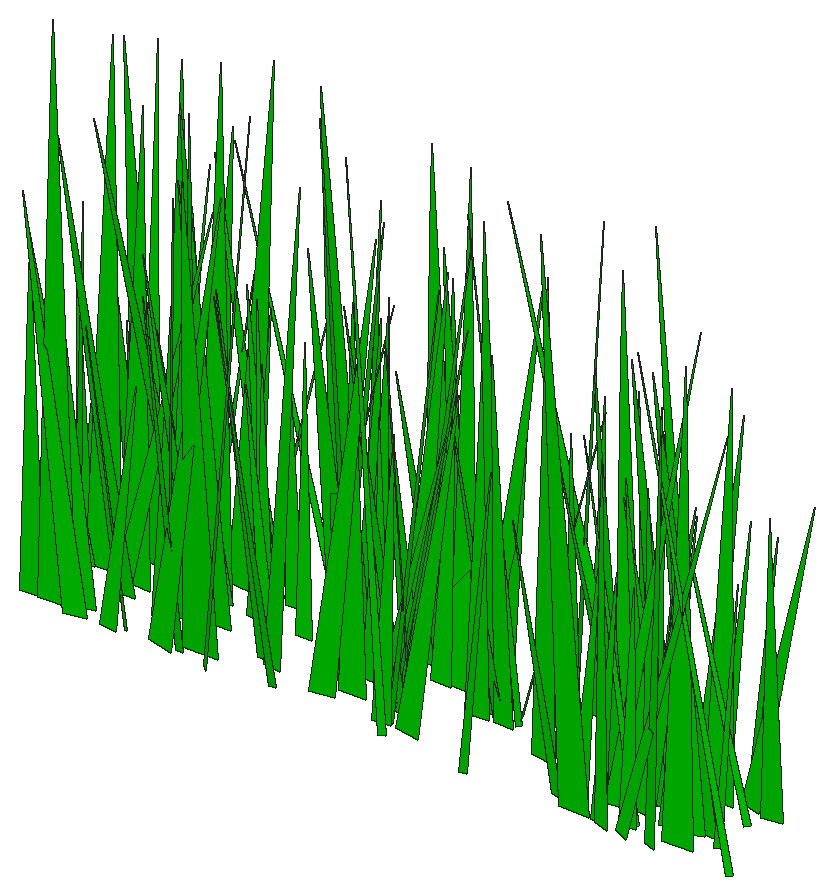
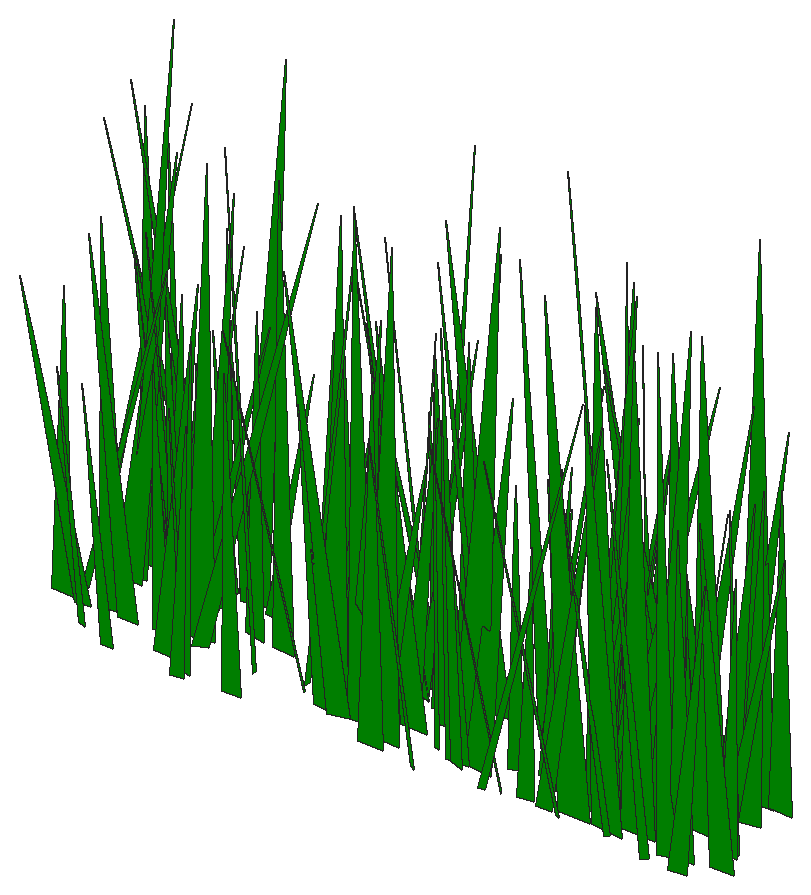
# SketchUp Ruby script. Lengths in inches.
U = 1.inch
M = Sketchup.active_model
def pt(a) = Geom::Point3d.new(a.map { |v| v * U })
def face(e, loops, mat)
  f = e.add_face(loops[0].map { |a| pt(a) })
  loops[1..].each { |l| e.add_face(l.map { |a| pt(a) }).erase! }
  f.material = f.back_material = mat if mat
  f
end
# faces: each face lists its corners as indices into pts; further lists are holes
def faces(e, pts, list, mat = nil) = list.each { |f| face(e, (f[0].is_a?(Array) ? f : [f]).map { |l| l.map { |i| pts[i] } }, mat) }
# xy, xz, yz: faces in a plane at the given z, y or x. An outline is a flat list of corners, or four numbers for a rectangle; further outlines are holes
def ring(l) = l.size == 4 ? [[l[0], l[1]], [l[2], l[1]], [l[2], l[3]], [l[0], l[3]]] : l.each_slice(2).to_a
def flat(e, list, mat, &to3) = list.each { |f| face(e, (f[0].is_a?(Array) ? f : [f]).map { |l| ring(l).map { |u, v| to3.(u, v) } }, mat) }
def xy(e, z, list, mat = nil) = flat(e, list, mat) { |x, y| [x, y, z] }
def xz(e, y, list, mat = nil) = flat(e, list, mat) { |x, z| [x, y, z] }
def yz(e, x, list, mat = nil) = flat(e, list, mat) { |y, z| [x, y, z] }
def lines(e, pts, list) = list.each { |a, b| e.add_line(pt(pts[a]), pt(pts[b])) }
# prism: a flat outline (further loops are holes) pulled along v
def prism(e, loops, v, mat = nil)
  f = face(e, loops, mat); d = Geom::Vector3d.new(v.map { |x| x * U })
  f.pushpull(f.normal.samedirection?(d) ? d.length : -d.length)
end
def box(e, o, s, mat = nil) = prism(e, [[o, [o[0] + s[0], o[1], o[2]], [o[0] + s[0], o[1] + s[1], o[2]], [o[0], o[1] + s[1], o[2]]]], [0, 0, s[2]], mat)
def at(x, y, z, deg = 0) = Geom::Transformation.translation(pt([x, y, z])) * Geom::Transformation.rotation(ORIGIN, Z_AXIS, deg.degrees)
def axes(o, x, y, z) = Geom::Transformation.new([*x, 0, *y, 0, *z, 0, *pt(o).to_a, 1])
def part(name) = M.definitions.add(name)
# library, detail: a bought-in or finely detailed component or shape, given as its bounding box
def library(name, o, s) = part(name).tap { |d| box(d.entities, o, s) }
def detail(e, o, s) = box(e.add_group.entities, o, s)
def put(e, d, t, mat = nil) = e.add_instance(d, t).tap { |i| i.material = mat if mat }
def group(e, t, mat = nil) = e.add_group.tap { |g| g.transformation = t; g.material = mat if mat }.entities
root = M.entities
M.materials.add("[Color G06]").color = [0, 204, 0]
c1 = part("fur_instance\#9")
p = [[0.8125,0,1.79],[0.67,-0.02,1.48],[0,-0.11,0],[0,0.11,0]]
faces(c1.entities,p,[[0,1,2,3]])
put(root,c1,axes([40.12,23.45,4.28],[-2.85245,0.30884,0.19412],[2.21845,0.39741,0.18428],[0.02687,-0.02469,5.39428]),"[Color G06]")
put(root,c1,axes([39.12,24.88,4.28],[0.44587,0.55522,0.43094],[3.99144,-0.06132,-0.15003],[0.06794,-0.04151,5.9861]),"[Color G06]")
put(root,c1,axes([39.53,24.09,4.28],[-1.47784,0.3217,1.91072],[2.58234,0.21807,0.24368],[0.53687,-0.16338,4.08752]),"[Color G06]")
put(root,c1,axes([39.44,23.875,4.28],[3.17546,0.17629,2.14393],[1.36851,-0.48036,0.0098],[-1.33536,-0.07307,5.10824]),"[Color G06]")
put(root,c1,axes([40.04,25.73,4.28],[-1.25995,-0.44632,0.01521],[-3.19526,0.17548,0.29333],[0.18635,-0.00871,5.13257]),"[Color G06]")
put(root,c1,axes([39.9375,21.28,4.28],[-0.04363,0.5128,0.83195],[3.71653,0.00302,0.22126],[-0.14312,-0.0778,5.49207]),"[Color G06]")
put(root,c1,axes([40.17,22.35,4.28],[-1.71212,0.49575,0.61747],[3.56156,0.2423,-0.28791],[0.35356,-0.04012,5.89045]),"[Color G06]")
put(root,c1,axes([40.41,25.09,4.28],[-0.2839,0.54186,0.38757],[3.8943,0.03985,-0.02844],[0.03791,-0.03587,5.82309]),"[Color G06]")
put(root,c1,axes([40.58,23.59,4.28],[0.53286,0.81064,0.81045],[5.83043,-0.07789,0.3865],[-0.30808,-0.07192,8.71631]),"[Color G06]")
put(root,c1,axes([41.58,21.08,4.28],[-2.68815,0.49164,0.54662],[3.54364,0.37426,0.25796],[0.08386,-0.05517,6.62131]),"[Color G06]")
put(root,c1,axes([40.51,24.95,4.28],[2.30914,0.16016,1.70391],[1.34151,-0.34437,-0.34264],[-0.9051,-0.10181,3.83924]),"[Color G06]")
put(root,c1,axes([40.79,21.3,4.28],[-1.94564,0.73172,3.76087],[5.76334,0.29356,0.09892],[0.80672,-0.3325,8.36373]),"[Color G06]")
put(root,c1,axes([41.96,22.81,4.28],[-3.36752,-0.46867,1.06526],[-3.42077,0.47034,-0.38423],[0.32011,0.09577,7.10044]),"[Color G06]")
put(root,c1,axes([41.54,21.58,4.28],[-1.2926,0.44884,0.766],[3.25907,0.1771,0.36367],[-0.03773,-0.07894,5.17128]),"[Color G06]")
put(root,c1,axes([40.85,25.21,4.28],[-4.35201,0.29976,3.63094],[2.42253,0.67732,0.06246],[2.15741,-0.15587,7.25434]),"[Color G06]")
put(root,c1,axes([41.42,24.6,4.28],[-1.33979,-0.77155,1.33619],[-5.5985,0.19029,0.08295],[0.26499,0.11932,8.50806]),"[Color G06]")
put(root,c1,axes([41.77,23.53,4.28],[2.11226,0.16366,1.89723],[1.30087,-0.33453,0.07983],[-1.13866,-0.0786,3.61063]),"[Color G06]")
put(root,c1,axes([41.76,23.4,4.28],[1.30253,-0.60335,3.45497],[-4.88502,-0.19005,0.30115],[-0.44897,0.31746,6.74666]),"[Color G06]")
put(root,c1,axes([41.25,25.7,4.28],[3.97968,-0.126,1.6751],[-0.96593,-0.57436,0.16321],[-1.06751,0.04999,6.09712]),"[Color G06]")
put(root,c1,axes([42.23,24.73,4.28],[-0.08104,0.74769,1.61282],[5.4693,0.01021,0.06995],[-0.03143,-0.15056,8.01433]),"[Color G06]")
put(root,c1,axes([43.875,23.49,4.28],[-4.07687,-0.46189,0.12276],[-3.31329,0.56845,-0.09246],[0.02473,0.01392,7.85025]),"[Color G06]")
put(root,c1,axes([43.18,21.29,4.28],[-3.05858,-0.00912,0.90232],[-0.11198,0.43336,-0.34468],[0.59685,0.03457,4.55931]),"[Color G06]")
put(root,c1,axes([43.03,25.13,4.28],[0.87527,0.70528,0.00052],[5.05312,-0.12194,0.32835],[-0.21654,0.00518,7.66451]),"[Color G06]")
put(root,c1,axes([42.7,21.1,4.28],[1.56069,-0.31586,0.71684],[-2.3132,-0.21616,0.30827],[-0.09896,0.07148,4.09956]),"[Color G06]")
put(root,c1,axes([41.72,22.92,4.28],[4.18376,-0.32444,0.21167],[-2.33055,-0.58297,0.24962],[-0.04249,0.02996,7.15043]),"[Color G06]")
put(root,c1,axes([44.04,24.15,4.28],[-3.04206,-0.4363,1.2577],[-3.15653,0.43539,0.2961],[0.73067,0.06443,6.51543]),"[Color G06]")
put(root,c1,axes([43.47,22.42,4.28],[1.61179,0.3871,1.23984],[2.83559,-0.23793,0.29931],[-0.59461,-0.08536,4.78818]),"[Color G06]")
put(root,c1,axes([44.375,24.09,4.28],[-1.61041,0.32888,0.22325],[2.36127,0.22291,0.32439],[-0.0955,-0.03424,4.25592]),"[Color G06]")
put(root,c1,axes([42.88,25.32,4.28],[3.32389,-0.08797,0.96952],[-0.64275,-0.47193,0.00294],[-0.63694,0.01714,5.05649]),"[Color G06]")
put(root,c1,axes([43.67,24.47,4.28],[-0.49846,0.74899,2.28351],[5.57775,0.07713,-0.18644],[0.27024,-0.21041,8.06001]),"[Color G06]")
put(root,c1,axes([44.63,22.85,4.28],[-2.74102,-0.16449,0.75095],[-1.23185,0.38373,-0.38792],[0.35573,0.06131,4.44303]),"[Color G06]")
put(root,c1,axes([43.84,22.76,4.28],[-1.16878,0.43335,2.18051],[3.37735,0.18371,-0.15035],[0.61619,-0.18494,4.96]),"[Color G06]")
put(root,c1,axes([44.93,22.38,4.28],[-2.90629,-0.38229,0.67175],[-2.76421,0.40699,-0.10738],[0.27729,0.05033,5.97027]),"[Color G06]")
put(root,c1,axes([45.21,25.22,4.28],[-3.96426,0.29588,1.18407],[2.18573,0.55814,0.3245],[0.59363,-0.07918,6.71235]),"[Color G06]")
put(root,c1,axes([44.68,23.26,4.28],[-3.70896,0.24437,1.80022],[1.75941,0.54231,-0.35953],[1.19429,-0.04002,6.12038]),"[Color G06]")
put(root,c1,axes([44.23,21.83,4.28],[-4.11597,-0.09811,2.95033],[-0.72754,0.63585,0.16175],[1.96532,0.02991,6.23875]),"[Color G06]")
put(root,c1,axes([44.93,23.04,4.28],[-2.52644,-0.63889,2.27151],[-4.80201,0.35702,-0.39511],[0.49189,0.20389,7.80968]),"[Color G06]")
put(root,c1,axes([45.01,21.31,4.28],[-3.27274,-0.18283,1.3921],[-1.39777,0.46901,-0.26419],[0.79555,0.07191,5.26266]),"[Color G06]")
put(root,c1,axes([44.25,25.07,4.28],[1.85243,0.73626,1.88589],[5.41345,-0.26442,-0.0193],[-0.40525,-0.16664,8.36277]),"[Color G06]")
put(root,c1,axes([44.79,22.05,4.28],[-4.66954,-0.25669,3.43881],[-2.07416,0.71337,-0.17439],[2.0929,0.13429,7.49963]),"[Color G06]")
put(root,c1,axes([44.42,21.21,4.28],[3.18828,0.53718,1.30508],[3.93312,-0.44618,-0.36599],[-0.36458,-0.11579,7.46465]),"[Color G06]")
put(root,c1,axes([47.26,25.42,4.28],[-4.91589,0.08106,0.36127],[0.59262,0.68538,0.34647],[0.21253,-0.03609,7.39023]),"[Color G06]")
put(root,c1,axes([45.53,21.57,4.28],[-0.16652,-0.77235,0.00783],[-5.53873,0.02322,0.00849],[0.00583,0.00071,8.28177]),"[Color G06]")
put(root,c1,axes([45.43,23.98,4.28],[2.38175,0.29892,1.42613],[2.21462,-0.34903,0.14227],[-0.77537,-0.07868,4.78705]),"[Color G06]")
put(root,c1,axes([46.21,23.76,4.28],[-2.2505,0.37025,1.19816],[2.7297,0.32117,0.05201],[0.49108,-0.08849,5.20173]),"[Color G06]")
put(root,c1,axes([45.94,25.11,4.28],[-1.16822,0.34539,1.05232],[2.55153,0.1698,-0.07516],[0.34726,-0.0857,4.09233]),"[Color G06]")
put(root,c1,axes([46.03,23.72,4.28],[-2.25727,0.32442,1.67701],[2.43983,0.33601,-0.13146],[0.84786,-0.10322,4.84301]),"[Color G06]")
put(root,c1,axes([44.64,25.33,4.28],[3.68565,0.12271,0.38905],[0.88593,-0.51496,-0.08893],[-0.23931,-0.01652,5.66261]),"[Color G06]")
put(root,c1,axes([47,22.39,4.28],[-3.36731,-0.21704,1.2149],[-1.62701,0.47786,-0.26638],[0.66045,0.0706,5.53792]),"[Color G06]")
put(root,c1,axes([46.59,23.0625,4.28],[0.27,-0.39209,1.36575],[-2.95249,-0.04246,-0.09639],[-0.1548,0.12591,4.22064]),"[Color G06]")
put(root,c1,axes([47.17,22.54,4.28],[-1.66988,0.31077,0.77043],[2.27575,0.23469,0.14356],[0.23075,-0.06566,4.1596]),"[Color G06]")
put(root,c1,axes([46.14,21.02,4.28],[5.69893,0.13608,2.64151],[1.04334,-0.83037,-0.11401],[-1.72843,-0.05256,8.64069]),"[Color G06]")
put(root,c1,axes([47.17,24,4.28],[1.91114,-0.27734,2.13718],[-2.2855,-0.29289,0.19915],[-0.88141,0.15811,4.11762]),"[Color G06]")
put(root,c1,axes([48.2,21.34,4.28],[-3.70295,-0.19382,1.03201],[-1.44498,0.52145,-0.33108],[0.56642,0.06314,5.90211]),"[Color G06]")
put(root,c1,axes([48.01,24.65,4.28],[-0.75998,-0.60579,0.19153],[-4.34378,0.10527,-0.25174],[-0.14392,0.02164,6.58663]),"[Color G06]")
put(root,c1,axes([47.55,22.14,4.28],[3.93587,0.41903,2.29981],[3.11444,-0.57787,0.18901],[-1.30302,-0.11549,7.3985]),"[Color G06]")
put(root,c1,axes([46.74,25.22,4.28],[3.75999,0.04929,0.42335],[0.34247,-0.52549,0.23363],[-0.29645,0.01807,5.63951]),"[Color G06]")
put(root,c1,axes([48.37,24.6,4.28],[-1.0832,-0.83788,1.06205],[-6.04963,0.15172,-0.03277],[0.10434,0.09806,9.12507]),"[Color G06]")
put(root,c1,axes([48.7,24.08,4.28],[-5.04094,-0.22111,2.62842],[-1.59717,0.74333,0.34092],[1.74818,0.04154,7.89062]),"[Color G06]")
put(root,c1,axes([48.65,24.82,4.28],[3.86213,0.30249,2.41646],[2.25592,-0.57698,0.24307],[-1.49351,-0.08929,6.61595]),"[Color G06]")
put(root,c1,axes([48.72,24.68,4.28],[1.23239,-0.48642,0.7673],[-3.5235,-0.17266,0.06723],[-0.12819,0.06961,5.52885]),"[Color G06]")
put(root,c1,axes([49.66,24.4,4.28],[-3.31285,-0.15227,2.41291],[-1.12798,0.51185,0.25122],[1.5895,0.04586,5.20728]),"[Color G06]")
put(root,c1,axes([49.14,23.02,4.28],[4.5547,0.22077,2.01328],[1.70523,-0.65555,-0.35945],[-1.18881,-0.09449,7.19788]),"[Color G06]")
put(root,c1,axes([50.17,22.34,4.28],[-0.06874,0.5647,1.44172],[4.1625,0.00737,0.11174],[-0.06047,-0.13465,6.05232]),"[Color G06]")
put(root,c1,axes([49.52,25.6875,4.28],[3.28467,0.11231,1.00551],[0.81818,-0.46711,0.02345],[-0.65722,-0.02018,5.05456]),"[Color G06]")
put(root,c1,axes([50.21,23.25,4.28],[1.3316,-0.52058,1.27764],[-3.82125,-0.18904,0.04802],[-0.25623,0.11381,5.92367]),"[Color G06]")
put(root,c1,axes([49.5,21.88,4.28],[3.817,-0.50031,1.12969],[-3.6229,-0.53805,-0.0299],[-0.56459,0.07014,7.82932]),"[Color G06]")
put(root,c1,axes([51.41,24.79,4.28],[-1.73515,-0.40131,0.02022],[-2.87789,0.24195,-0.02453],[-0.00707,0.0028,5.02244]),"[Color G06]")
put(root,c1,axes([51.23,23.65,4.28],[-0.85631,-0.47007,0.62233],[-3.39621,0.1176,-0.23426],[-0.05059,0.06164,5.19289]),"[Color G06]")
put(root,c1,axes([50.99,22.61,4.28],[-1.49738,0.34444,1.11468],[2.52223,0.22075,-0.26744],[0.54392,-0.0754,4.30878]),"[Color G06]")
put(root,c1,axes([51.85,22.35,4.28],[-3.52163,-0.30445,1.11288],[-2.244,0.49604,-0.27293],[0.53448,0.07665,6.18675]),"[Color G06]")
put(root,c1,axes([51.16,24.99,4.28],[-0.28699,0.73119,2.39369],[5.48041,0.03181,0.35136],[-0.15798,-0.22465,7.84073]),"[Color G06]")
put(root,c1,axes([51.22,25.42,4.28],[-0.39201,0.55416,1.30054],[4.06789,0.05494,0.04973],[0.05153,-0.12122,5.96814]),"[Color G06]")
put(root,c1,axes([50.85,23.94,4.28],[1.48248,0.60516,0.65009],[4.3605,-0.207,-0.07612],[-0.09219,-0.0597,6.85363]),"[Color G06]")
put(root,c1,axes([52.17,21.11,4.28],[-5.64778,0.07935,2.74293],[0.54179,0.82809,-0.26007],[1.84349,-0.00027,8.47977]),"[Color G06]")
put(root,c1,axes([51.67,24.31,4.28],[0.38428,0.44524,0.26178],[3.19714,-0.05396,0.05911],[-0.06025,-0.02359,4.8061]),"[Color G06]")
put(root,c1,axes([51.74,21.64,4.28],[0.81675,0.43423,0.31541],[3.10847,-0.11591,0.35038],[-0.28065,-0.02008,4.79871]),"[Color G06]")
put(root,c1,axes([52.42,24.42,4.28],[-2.21811,0.57653,0.81919],[4.14958,0.31376,-0.26902],[0.41863,-0.05535,7.00722]),"[Color G06]")
put(root,c1,axes([52.53,21.96,4.28],[-3.7146,-0.03906,1.80542],[-0.25999,0.54468,0.15894],[1.21248,-0.00288,5.56524]),"[Color G06]")
put(root,c1,axes([52.23,24.56,4.28],[3.60088,-0.52964,2.80257],[-3.98772,-0.5396,-0.26961],[-1.42842,0.17126,7.81761]),"[Color G06]")
put(root,c1,axes([51.33,21.98,4.28],[2.925,0.24264,0.2285],[1.74536,-0.40765,-0.17867],[-0.07013,-0.02523,5.08356]),"[Color G06]")
put(root,c1,axes([51.89,21.85,4.28],[4.52132,0.15562,1.72882],[1.12501,-0.65033,0.15262],[-1.14797,-0.0244,6.95858]),"[Color G06]")
put(root,c1,axes([51.53,22.44,4.28],[4.38594,0.08941,0.90018],[0.65849,-0.61687,-0.12836],[-0.58331,-0.02411,6.62353]),"[Color G06]")
put(root,c1,axes([51.74,22.64,4.28],[4.79065,0.25143,1.54673],[1.86221,-0.68014,-0.18341],[-0.92419,-0.06716,7.6481]),"[Color G06]")
put(root,c1,axes([52.66,21.6,4.28],[1.70611,0.49835,0.35546],[3.58086,-0.23651,-0.30039],[0.07938,-0.04199,5.91116]),"[Color G06]")
put(root,c1,axes([54.23,23.62,4.28],[-2.5369,-0.25198,0.62255],[-1.83075,0.356,-0.11186],[0.29536,0.04227,4.65378]),"[Color G06]")
put(root,c1,axes([53.78,23.85,4.28],[-2.15638,-0.62838,2.38413],[-4.69259,0.32479,0.35292],[0.9114,0.18551,7.458]),"[Color G06]")
put(root,c1,axes([53.55,23.5,4.28],[1.23385,-0.48803,1.20071],[-3.57186,-0.17897,-0.15737],[-0.36861,0.10062,5.54403]),"[Color G06]")
put(root,c1,axes([54.76,23.8,4.28],[-5.08559,0.0381,1.95962],[0.2616,0.73235,-0.11911],[1.31352,0.00165,7.61081]),"[Color G06]")
put(root,c1,axes([52.94,24.7,4.28],[3.46232,-0.44249,0.97066],[-3.21479,-0.48564,0.18287],[-0.39517,0.07387,7.01685]),"[Color G06]")
put(root,c1,axes([53.65,24.58,4.28],[-1.68176,-0.29221,2.7923],[-2.55613,0.28497,-0.01315],[1.16101,0.20412,4.01578]),"[Color G06]")
put(root,c1,axes([54.42,23.57,4.28],[-2.04181,-0.41712,2.03423],[-3.20714,0.30167,-0.08478],[0.7172,0.1615,5.41221]),"[Color G06]")
put(root,c1,axes([55.18,20.87,4.28],[2.80446,0.21722,1.16796],[1.54558,-0.40539,0.3711],[-0.8052,-0.0216,4.78026]),"[Color G06]")
put(root,c1,axes([54.56,24.1875,4.28],[3.8622,0.02817,0.20117],[0.20666,-0.53854,-0.19842],[-0.12739,-0.01948,5.77682]),"[Color G06]")
put(root,c1,axes([58.4,24.01,4.28],[-5.50729,0.28867,0.06226],[2.06973,0.76797,-0.08211],[0.05832,0.00513,8.79296]),"[Color G06]")
put(root,c1,axes([56.07,25.56,4.28],[1.63701,-0.398,1.55176],[-2.98581,-0.24101,-0.06527],[-0.55623,0.1224,4.9172]),"[Color G06]")
put(root,c1,axes([56.42,22.79,4.28],[3.06988,0.48795,3.09743],[3.85387,-0.46469,-0.12257],[-1.29905,-0.22546,6.95614]),"[Color G06]")
put(root,c1,axes([56.32,24.22,4.28],[5.29806,0.00443,2.70238],[0.04696,-0.7806,-0.05858],[-1.8078,-0.00729,7.91827]),"[Color G06]")
put(root,c1,axes([57.96,21.43,4.28],[-2.25329,-0.25741,0.4088],[-1.84874,0.31606,0.09971],[0.254,0.01694,4.35237]),"[Color G06]")
put(root,c1,axes([57.57,22.62,4.28],[-1.6751,-0.37021,2.59735],[-3.0995,0.24957,-0.37873],[0.67936,0.22583,4.67637]),"[Color G06]")
put(root,c1,axes([57.86,25.74,4.28],[1.71283,-0.23213,2.16536],[-1.97331,-0.2756,0.09271],[-0.98805,0.14801,3.56859]),"[Color G06]")
put(root,c1,axes([57.86,25.44,4.28],[-2.68409,-0.28082,2.06488],[-2.19198,0.40324,-0.06486],[1.07686,0.12085,5.01476]),"[Color G06]")
put(root,c1,axes([57.97,25.35,4.28],[2.61411,-0.05031,1.39109],[-0.40729,-0.38592,0.10643],[-0.91136,0.02817,3.94258]),"[Color G06]")
put(root,c1,axes([58.875,21.03,4.28],[2.6675,0.61688,4.62567],[5.09312,-0.44725,0.29108],[-1.79146,-0.35298,7.71523]),"[Color G06]")
put(root,c1,axes([58.89,24.97,4.28],[-1.80829,-0.51777,1.23184],[-3.79301,0.2549,-0.1297],[0.28124,0.10871,6.17117]),"[Color G06]")
put(root,c1,axes([59.69,22.42,4.28],[-3.07598,-0.25526,0.33393],[-1.84282,0.42774,-0.35732],[0.06907,0.0446,5.33781]),"[Color G06]")
put(root,c1,axes([58.7,23.65,4.28],[-2.80134,0.57613,2.47341],[4.31829,0.41786,-0.25623],[1.07767,-0.17676,7.45615]),"[Color G06]")
put(root,c1,axes([59.63,22.09,4.28],[-2.94182,-0.46645,1.79864],[-3.43055,0.42961,0.26531],[0.9322,0.10898,6.65248]),"[Color G06]")
put(root,c1,axes([60.11,23.5,4.28],[-2.39493,0.26591,0.31378],[1.91018,0.33487,-0.03296],[0.17801,-0.01582,4.57535]),"[Color G06]")
put(root,c1,axes([58.87,21.23,4.28],[1.35024,-0.36286,0.25547],[-2.60599,-0.18875,-0.03087],[-0.09709,0.01983,4.38145]),"[Color G06]")
put(root,c1,axes([60.1,22.62,4.28],[1.30122,-0.33756,2.92142],[-2.9303,-0.23228,-0.16773],[-1.046,0.23079,4.10412]),"[Color G06]")
put(root,c1,axes([60.68,21.46,4.28],[-3.8814,0.08673,1.19677],[0.66588,0.55121,0.23497],[0.76464,-0.03975,5.87035]),"[Color G06]")
put(root,c1,axes([59.93,20.875,4.28],[2.91322,0.27226,2.49284],[2.22342,-0.44341,-0.24089],[-1.2847,-0.15003,5.2359]),"[Color G06]")
put(root,c1,axes([59.82,23.99,4.28],[1.20053,-0.34282,1.26074],[-2.57699,-0.17388,0.0499],[-0.33872,0.10783,4.08875]),"[Color G06]")
put(root,c1,axes([59.7,23.37,4.28],[2.31997,-0.35335,1.14489],[-2.55028,-0.33641,-0.38346],[-0.70972,0.05381,5.12036]),"[Color G06]")
put(root,c1,axes([59.71,21.03,4.28],[-1.41524,0.24728,2.38776],[2.14318,0.24565,-0.08495],[1.05059,-0.16802,3.38983]),"[Color G06]")
put(root,c1,axes([60.32,22.71,4.28],[0.51969,-0.4775,0.79338],[-3.45656,-0.07672,-0.24639],[-0.24445,0.06961,5.1706]),"[Color G06]")
put(root,c1,axes([60.5,21.3,4.28],[0.2366,0.3753,0.04648],[2.68916,-0.03315,0.16708],[-0.11409,-0.00295,4.03455]),"[Color G06]")
put(root,c1,axes([60.47,25.61,4.28],[2.25281,-0.227,0.67404],[-1.62229,-0.31996,-0.26672],[-0.47068,0.01632,4.14547]),"[Color G06]")
put(root,c1,axes([59.42,22,4.28],[5.33549,-0.20978,1.122],[-1.53968,-0.74957,0.25543],[-0.6754,0.05154,8.28126]),"[Color G06]")
put(root,c1,axes([60.54,22.19,4.28],[3.7527,-0.02011,1.42709],[-0.08411,-0.53906,-0.37876],[-0.96201,-0.03133,5.60003]),"[Color G06]")
put(root,c1,axes([60.42,22.14,4.28],[2.37947,-0.40437,0.36353],[-2.9098,-0.33006,0.36839],[0.03699,0.04801,5.59424]),"[Color G06]")
put(root,c1,axes([60.91,24.1,4.28],[2.28216,0.47326,1.30969],[3.48846,-0.32089,-0.25826],[-0.3419,-0.11506,6.10708]),"[Color G06]")
put(root,c1,axes([63.01,23.37,4.28],[-4.01386,0.10206,0.28186],[0.73586,0.56014,0.10783],[0.17254,-0.01462,6.09697]),"[Color G06]")
put(root,c1,axes([62.22,22.07,4.28],[-5.40437,0.3567,2.8778],[2.71996,0.7894,0.16989],[1.68899,-0.1299,8.9347]),"[Color G06]")
put(root,c1,axes([61.56,23.92,4.28],[-0.08495,0.62439,0.85667],[4.51235,0.01405,-0.17697],[0.13022,-0.07957,6.69111]),"[Color G06]")
put(root,c1,axes([62.34,22.29,4.28],[-2.09129,-0.63401,0.69588],[-4.56737,0.29252,-0.04528],[0.16692,0.06076,7.47952]),"[Color G06]")
put(root,c1,axes([61.24,22,4.28],[3.10995,-0.17952,1.22843],[-1.32714,-0.4463,0.01295],[-0.75602,0.04499,5.03053]),"[Color G06]")
put(root,c1,axes([61.65,20.84,4.28],[3.987,0.23962,2.58265],[1.86188,-0.59762,-0.05106],[-1.5723,-0.10008,6.48854]),"[Color G06]")
put(root,c1,axes([61.79,25.07,4.28],[2.40197,0.17192,0.946],[1.23295,-0.34574,0.22481],[-0.63278,-0.02107,4.02892]),"[Color G06]")
put(root,c1,axes([62.25,21.3,4.28],[1.27004,0.66648,1.94585],[4.92667,-0.18949,0.27308],[-0.51673,-0.16858,7.38622]),"[Color G06]")
put(root,c1,axes([60.64,20.85,4.28],[4.53374,0.29006,0.22877],[2.08504,-0.6316,-0.30869],[-0.05283,-0.03508,7.44875]),"[Color G06]")
put(root,c1,axes([64.34,20.92,4.28],[-5.32115,0.07522,0.9131],[0.53178,0.74687,-0.1457],[0.61762,0.00502,7.99228]),"[Color G06]")
put(root,c1,axes([63.35,23.99,4.28],[0.7619,-0.46958,0.43816],[-3.37228,-0.10847,-0.25573],[-0.2321,0.03454,5.15387]),"[Color G06]")
put(root,c1,axes([62.47,24.17,4.28],[2.22983,0.4025,0.20176],[2.88725,-0.30938,-0.37603],[0.11691,-0.03632,5.43837]),"[Color G06]")
put(root,c1,axes([63.14,21.93,4.28],[2.64231,-0.13642,1.14067],[-0.96594,-0.38331,-0.2682],[-0.77883,0.01257,4.20258]),"[Color G06]")
